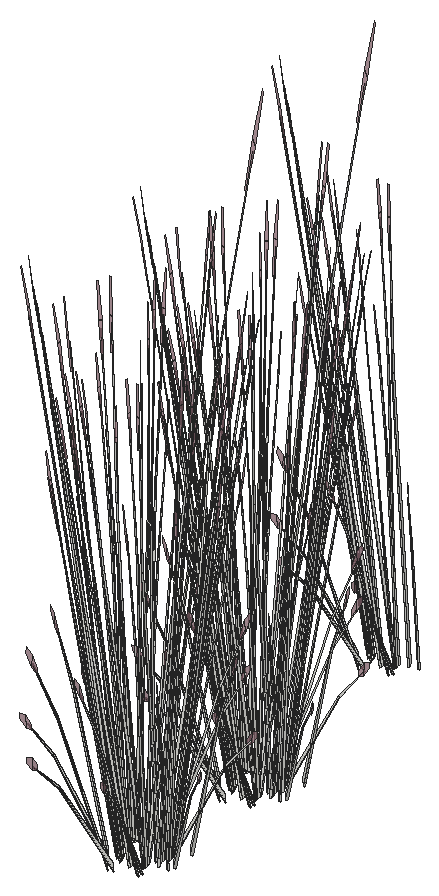
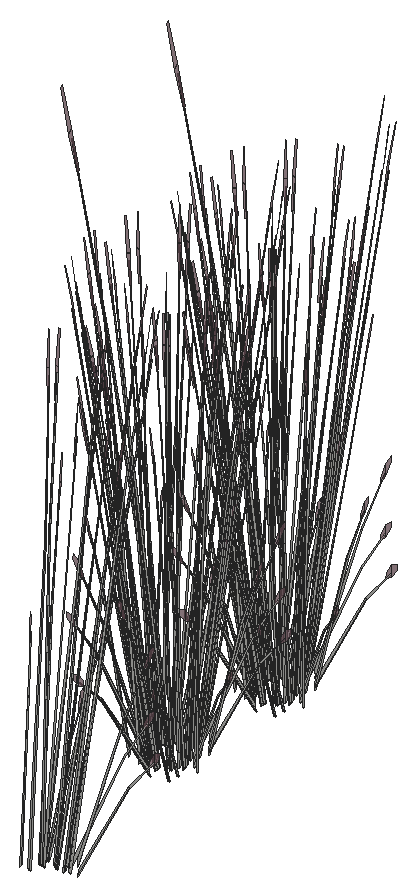
# SketchUp Ruby script. Lengths in inches.
U = 1.inch
M = Sketchup.active_model
def pt(a) = Geom::Point3d.new(a.map { |v| v * U })
def face(e, loops, mat)
  f = e.add_face(loops[0].map { |a| pt(a) })
  loops[1..].each { |l| e.add_face(l.map { |a| pt(a) }).erase! }
  f.material = f.back_material = mat if mat
  f
end
# faces: each face lists its corners as indices into pts; further lists are holes
def faces(e, pts, list, mat = nil) = list.each { |f| face(e, (f[0].is_a?(Array) ? f : [f]).map { |l| l.map { |i| pts[i] } }, mat) }
# xy, xz, yz: faces in a plane at the given z, y or x. An outline is a flat list of corners, or four numbers for a rectangle; further outlines are holes
def ring(l) = l.size == 4 ? [[l[0], l[1]], [l[2], l[1]], [l[2], l[3]], [l[0], l[3]]] : l.each_slice(2).to_a
def flat(e, list, mat, &to3) = list.each { |f| face(e, (f[0].is_a?(Array) ? f : [f]).map { |l| ring(l).map { |u, v| to3.(u, v) } }, mat) }
def xy(e, z, list, mat = nil) = flat(e, list, mat) { |x, y| [x, y, z] }
def xz(e, y, list, mat = nil) = flat(e, list, mat) { |x, z| [x, y, z] }
def yz(e, x, list, mat = nil) = flat(e, list, mat) { |y, z| [x, y, z] }
def lines(e, pts, list) = list.each { |a, b| e.add_line(pt(pts[a]), pt(pts[b])) }
# prism: a flat outline (further loops are holes) pulled along v
def prism(e, loops, v, mat = nil)
  f = face(e, loops, mat); d = Geom::Vector3d.new(v.map { |x| x * U })
  f.pushpull(f.normal.samedirection?(d) ? d.length : -d.length)
end
def box(e, o, s, mat = nil) = prism(e, [[o, [o[0] + s[0], o[1], o[2]], [o[0] + s[0], o[1] + s[1], o[2]], [o[0], o[1] + s[1], o[2]]]], [0, 0, s[2]], mat)
def at(x, y, z, deg = 0) = Geom::Transformation.translation(pt([x, y, z])) * Geom::Transformation.rotation(ORIGIN, Z_AXIS, deg.degrees)
def axes(o, x, y, z) = Geom::Transformation.new([*x, 0, *y, 0, *z, 0, *pt(o).to_a, 1])
def part(name) = M.definitions.add(name)
# library, detail: a bought-in or finely detailed component or shape, given as its bounding box
def library(name, o, s) = part(name).tap { |d| box(d.entities, o, s) }
def detail(e, o, s) = box(e.add_group.entities, o, s)
def put(e, d, t, mat = nil) = e.add_instance(d, t).tap { |i| i.material = mat if mat }
def group(e, t, mat = nil) = e.add_group.tap { |g| g.transformation = t; g.material = mat if mat }.entities
root = M.entities
M.materials.add("LightPink_Translucent").color = [144, 107, 117]
M.materials["LightPink_Translucent"].alpha = 0.75
c1 = part("blade")
p = [[2.15,0.21,22],[0,0.17,0],[0.09,0.45,0],[2.18,0.31,22],[2.29,0.31,22],[0.38,0.45,0],
  [2.48,0.24,33],[2.49,0.24,33],[2.48,0.22,33]]
faces(c1.entities,p,[[0,1,2,3],[4,5,2,3],[6,3,4,7],[8,0,3,6]])
c2 = part("seeds")
p = [[0.3,-0.1,1.38],[-0.01,-0.03,1.59],[-0.01,-0.03,0.03],[0.14,-0.07,-0.07],[0.29,-0.03,3],[0.15,0.01,3.11]]
faces(c2.entities,p,[[0,1,2,3],[1,0,4,5]],"LightPink_Translucent")
c3 = part("blade with seeds")
put(c3.entities,c1,at(0,0,0))
put(c3.entities,c2,axes([2.4,0.25,30.99],[1.5799,-0.05474,1.17369],[-0.12525,1.92788,0.29478],[-0.07173,-0.02425,1.56792]))
put(root,c3,axes([401.89,8.58,4.72],[-0.05398,-0.06539,1.74944],[-0.36026,0.04145,-0.27667],[-0.0575,-0.15639,0.14031]))
put(root,c3,axes([403.51,9.38,4.72],[-0.00341,-0.09282,1.74944],[-0.28775,-0.26825,-0.27667],[0.04449,-0.16261,0.14031]))
put(root,c3,axes([403.43,9.05,4.71],[-0.03584,0.03562,1.77383],[-0.35118,-0.12018,-0.16761],[-0.01271,-0.15545,0.31391]))
put(root,c3,axes([401.52,8.37,4.71],[-0.00658,0.0559,1.77383],[-0.32474,0.20287,-0.16761],[-0.09556,-0.1037,0.31391]))
put(root,c3,axes([401.45,9.36,5.09],[0.39316,-0.11987,0.53763],[0.06823,0.47021,0.4433],[-0.09247,-0.13858,1.11249]))
put(root,c3,axes([402.34,9.45,4.73],[0.34777,0.12192,0.48003],[-0.11892,0.40083,0.3958],[-0.0209,-0.15763,0.9933]))
put(root,c3,axes([402.4375,9.59,5.03],[-0.34538,0.21713,-0.1216],[-0.16972,-0.38536,-0.67495],[-0.04557,-0.16239,1.02557]))
put(root,c3,axes([403.15,10.08,5.03],[-0.3879,-0.02311,-0.1216],[0.0106,-0.43749,-0.67495],[0.02694,-0.1685,1.02557]))
put(root,c3,axes([402.43,9.42,4.73],[0.26007,-0.1585,0.0643],[0.12729,0.28902,0.50621],[-0.02512,-0.1274,0.77189]))
put(root,c3,axes([401.54,9.46,4.73],[0.16041,-0.29625,0.0643],[0.22843,0.17248,0.50621],[-0.07385,-0.09498,0.77189]))
put(root,c3,axes([402.33,9.74,5.05],[-0.1064,0.35863,0.35414],[-0.31043,-0.1046,-0.4572],[-0.02846,-0.14439,0.87481]))
put(root,c3,axes([403.125,9.89,4.73],[0.25132,0.3182,0.48003],[-0.2669,0.27442,0.3958],[0.04636,-0.14929,0.9933]))
put(root,c3,axes([401.61,9.43,5.43],[-0.23555,0.44708,-0.13619],[-0.34112,-0.25757,-0.75594],[-0.11858,-0.12631,1.14864]))
put(root,c3,axes([403.22,9.92,4.73],[0.29004,0.02173,0.0643],[-0.00795,0.32812,0.50621],[0.03035,-0.12569,0.77189]))
put(root,c3,axes([403,10.14,5.05],[-0.23881,0.24554,0.35414],[-0.22606,-0.28036,-0.4572],[0.0344,-0.14245,0.87481]))
put(root,c3,axes([400.71,9.3,4.72],[-0.07594,-0.00329,1.74944],[-0.24177,0.32918,-0.27667],[-0.129,-0.06726,0.14031]))
put(root,c3,axes([403.58,10.9375,5.03],[-0.32648,-0.25715,-0.1216],[0.18809,-0.3724,-0.67495],[0.09224,-0.12945,1.02557]))
put(root,c3,axes([401.59,9.8,5.05],[0.05451,0.37564,0.35414],[-0.31161,0.09919,-0.4572],[-0.0837,-0.10765,0.87481]))
put(root,c3,axes([400.65,10.04,5.09],[0.29147,-0.34417,0.53763],[0.25138,0.3655,0.4433],[-0.13675,-0.06349,1.11249]))
put(root,c3,axes([404.38,10.83,4.71],[-0.0461,-0.00354,1.77383],[-0.19143,-0.37951,-0.16761],[0.07688,-0.12478,0.31391]))
put(root,c3,axes([400.78,10.04,4.73],[0.01777,-0.35463,0.0643],[0.26836,0.00972,0.50621],[-0.1028,-0.03711,0.77189]))
put(root,c3,axes([403.42,10.9,5.05],[-0.30722,0.06665,0.35414],[-0.08112,-0.381,-0.4572],[0.08804,-0.10234,0.87481]))
put(root,c3,axes([403.7,10.84,4.73],[0.2423,0.19613,0.0643],[-0.14107,0.2793,0.50621],[0.07768,-0.0903,0.77189]))
put(root,c3,axes([403.63,10.76,4.73],[0.08753,0.42921,0.48003],[-0.34336,0.07449,0.3958],[0.1012,-0.10094,0.9933]))
put(root,c3,axes([404.55,11.28,4.72],[0.04898,-0.07104,1.74944],[-0.06269,-0.43574,-0.27667],[0.12289,-0.08262,0.14031]))
put(root,c3,axes([400.42,9.58,4.71],[0.02617,0.04654,1.77383],[-0.12614,0.41836,-0.16761],[-0.12775,0.00303,0.31391]))
put(root,c3,axes([400.97,10.31,5.05],[0.20082,0.29199,0.35414],[-0.2293,0.2764,-0.4572],[-0.1165,-0.04206,0.87481]))
put(root,c3,axes([400.91,10.12,5.03],[-0.0189,0.47427,-0.1216],[-0.35781,-0.01296,-0.67495],[-0.13781,-0.03295,1.02557]))
put(root,c3,axes([403.59,11.94,5.03],[-0.17758,-0.42229,-0.1216],[0.31518,-0.20752,-0.67495],[0.13282,-0.05572,1.02557]))
put(root,c3,axes([403.47,11.81,5.05],[-0.29332,-0.1301,0.35414],[0.08555,-0.37955,-0.4572],[0.11809,-0.0348,0.87481]))
put(root,c3,axes([400.4,11.12,4.73],[0.09971,-0.42522,0.48003],[0.32782,0.1454,0.3958],[-0.12892,0.02555,0.9933]))
put(root,c3,axes([400.37,11.01,4.73],[-0.12963,-0.31798,0.0643],[0.23638,-0.15564,0.50621],[-0.1042,0.03071,0.77189]))
put(root,c3,axes([403.73,11.93,4.73],[0.12963,0.31798,0.0643],[-0.23638,0.15564,0.50621],[0.1042,-0.03071,0.77189]))
put(root,c3,axes([403.71,11.82,4.73],[-0.09971,0.42522,0.48003],[-0.32782,-0.1454,0.3958],[0.12892,-0.02555,0.9933]))
put(root,c3,axes([400.64,11.125,5.05],[0.29332,0.1301,0.35414],[-0.08555,0.37955,-0.4572],[-0.11809,0.0348,0.87481]))
put(root,c3,axes([404.3,13.2,4.71],[-0.03191,-0.04083,1.77383],[0.06981,-0.43764,-0.16761],[0.12571,-0.02796,0.31391]))
put(root,c3,axes([400.14,11.42,4.72],[-0.05763,0.06055,1.74944],[0.0049,0.44239,-0.27667],[-0.13211,0.05753,0.14031]))
put(root,c3,axes([400.51,11,5.03],[0.17758,0.42229,-0.1216],[-0.31518,0.20752,-0.67495],[-0.13282,0.05572,1.02557]))
put(root,c3,axes([403.19,12.82,5.03],[0.0189,-0.47427,-0.1216],[0.35781,0.01296,-0.67495],[0.13781,0.03295,1.02557]))
put(root,c3,axes([403.14,12.63,5.05],[-0.20082,-0.29199,0.35414],[0.2293,-0.2764,-0.4572],[0.1165,0.04206,0.87481]))
put(root,c3,axes([403.5,12.53,4.72],[0.07571,-0.00789,1.74944],[0.20767,-0.36231,-0.27667],[0.13467,0.04783,0.14031]))
put(root,c3,axes([400.47,12.18,4.73],[-0.08753,-0.42921,0.48003],[0.34336,-0.07449,0.3958],[-0.1012,0.10094,0.9933]))
put(root,c3,axes([400.41,12.1,4.73],[-0.2423,-0.19613,0.0643],[0.14107,-0.2793,0.50621],[-0.07768,0.0903,0.77189]))
put(root,c3,axes([400.6875,12.04,5.05],[0.30722,-0.06665,0.35414],[0.08112,0.381,-0.4572],[-0.08804,0.10234,0.87481]))
put(root,c3,axes([399.5,11.87,4.71],[0.04504,0.01251,1.77383],[0.13934,0.41205,-0.16761],[-0.0922,0.10815,0.31391]))
put(root,c3,axes([403.32,12.9,4.73],[-0.01777,0.35463,0.0643],[-0.26836,-0.00972,0.50621],[0.1028,0.03711,0.77189]))
put(root,c3,axes([403.34,12.79,4.73],[-0.26024,0.30729,0.48003],[-0.22444,-0.32634,0.3958],[0.1221,0.05668,0.9933]))
put(root,c3,axes([399.99,13.12,5.65],[0.31145,0.12449,-0.06488],[-0.0958,0.38314,-0.29416],[-0.05094,0.05817,0.97024]))
put(root,c3,axes([402.52,13.14,5.05],[-0.05451,-0.37564,0.35414],[0.31161,-0.09919,-0.4572],[0.0837,0.10765,0.87481]))
put(root,c3,axes([402.72,10.98,4.47],[-0.30498,-0.24231,1.38283],[0.32203,-0.37727,0.59665],[0.0984,0.22736,1.33663]))
put(root,c3,axes([400.53,12,5.03],[0.32648,0.25715,-0.1216],[-0.18809,0.3724,-0.67495],[-0.09224,0.12945,1.02557]))
put(root,c3,axes([402.49,13.34,5.03],[0.21031,-0.39918,-0.1216],[0.30457,0.22997,-0.67495],[0.10587,0.11278,1.02557]))
put(root,c3,axes([401.1,12.8,5.05],[0.23881,-0.24554,0.35414],[0.22606,0.28036,-0.4572],[-0.0344,0.14245,0.87481]))
put(root,c3,axes([402.21,13.67,4.71],[0.00104,-0.05646,1.77383],[0.30246,-0.2491,-0.16761],[0.10506,0.08891,0.31391]))
put(root,c3,axes([400.88,13.02,4.73],[-0.29004,-0.02173,0.0643],[0.00795,-0.32812,0.50621],[-0.03035,0.12569,0.77189]))
put(root,c3,axes([400.98,13.05,4.73],[-0.25132,-0.3182,0.48003],[0.2669,-0.27442,0.3958],[-0.04636,0.14929,0.9933]))
put(root,c3,axes([401.77,13.2,5.05],[0.1064,-0.35863,0.35414],[0.31043,0.1046,-0.4572],[0.02846,0.14439,0.87481]))
put(root,c3,axes([402.56,13.48,4.73],[-0.16041,0.29625,0.0643],[-0.22843,-0.17248,0.50621],[0.07385,0.09498,0.77189]))
put(root,c3,axes([402.1875,14.48,5.65],[0.2439,-0.26754,-0.06488],[0.22348,0.29302,-0.29416],[0.01573,0.08303,0.97024]))
put(root,c3,axes([402.63,13.4,4.73],[-0.35104,0.10702,0.48003],[-0.06092,-0.41983,0.3958],[0.08256,0.12373,0.9933]))
put(root,c3,axes([401.67,13.53,4.73],[-0.26007,0.1585,0.0643],[-0.12729,-0.28902,0.50621],[0.02512,0.1274,0.77189]))
put(root,c3,axes([400.15,13.07,4.72],[-0.00877,0.09229,1.74944],[0.24897,0.32105,-0.27667],[-0.06518,0.15182,0.14031]))
put(root,c3,axes([400.95,12.86,5.4],[0.3879,0.02311,-0.13498],[-0.0106,0.43749,-0.74919],[-0.02694,0.1685,1.13838]))
put(root,c3,axes([401.67,13.35,5.03],[0.34538,-0.21713,-0.1216],[0.16972,0.38536,-0.67495],[0.04557,0.16239,1.02557]))
put(root,c3,axes([401.77,13.49,5.0625],[-0.34777,-0.12192,0.53283],[0.11892,-0.40083,0.43934],[0.0209,0.15763,1.10256]))
put(root,c3,axes([401.89,19.52,4.72],[-0.05398,-0.06539,1.74944],[-0.36026,0.04145,-0.27667],[-0.0575,-0.15639,0.14031]))
put(root,c3,axes([400.125,14.02,4.71],[0.04004,-0.02816,1.77383],[0.33095,0.18728,-0.16761],[-0.00778,0.15594,0.31391]))
put(root,c3,axes([403.51,20.33,4.72],[-0.00341,-0.09282,1.74944],[-0.28775,-0.26825,-0.27667],[0.04449,-0.16261,0.14031]))
put(root,c3,axes([403.43,19.99,4.71],[-0.03584,0.03562,1.77383],[-0.35118,-0.12018,-0.16761],[-0.01271,-0.15545,0.31391]))
put(root,c3,axes([401.58,14.21,4.72],[0.04474,0.0751,1.74944],[0.36104,0.0295,-0.27667],[0.03631,0.16562,0.14031]))
put(root,c3,axes([401.52,19.31,4.71],[-0.00658,0.0559,1.77383],[-0.32474,0.20287,-0.16761],[-0.09556,-0.1037,0.31391]))
put(root,c3,axes([401.45,20.3,5.09],[0.39316,-0.11987,0.53763],[0.06823,0.47021,0.4433],[-0.09247,-0.13858,1.11249]))
put(root,c3,axes([402.34,20.39,4.73],[0.34777,0.12192,0.48003],[-0.11892,0.40083,0.3958],[-0.0209,-0.15763,0.9933]))
put(root,c3,axes([402.4375,20.53,5.03],[-0.34538,0.21713,-0.1216],[-0.16972,-0.38536,-0.67495],[-0.04557,-0.16239,1.02557]))
put(root,c3,axes([403.15,21.02,5.03],[-0.3879,-0.02311,-0.1216],[0.0106,-0.43749,-0.67495],[0.02694,-0.1685,1.02557]))
put(root,c3,axes([402.43,20.36,4.73],[0.26007,-0.1585,0.0643],[0.12729,0.28902,0.50621],[-0.02512,-0.1274,0.77189]))
put(root,c3,axes([401.54,20.4,4.73],[0.16041,-0.29625,0.0643],[0.22843,0.17248,0.50621],[-0.07385,-0.09498,0.77189]))
put(root,c3,axes([402.33,20.68,5.05],[-0.1064,0.35863,0.35414],[-0.31043,-0.1046,-0.4572],[-0.02846,-0.14439,0.87481]))
put(root,c3,axes([403.125,20.84,4.73],[0.25132,0.3182,0.48003],[-0.2669,0.27442,0.3958],[0.04636,-0.14929,0.9933]))
put(root,c3,axes([401.61,20.375,5.43],[-0.23555,0.44708,-0.13619],[-0.34112,-0.25757,-0.75594],[-0.11858,-0.12631,1.14864]))
put(root,c3,axes([403.22,20.87,4.73],[0.29004,0.02173,0.0643],[-0.00795,0.32812,0.50621],[0.03035,-0.12569,0.77189]))
put(root,c3,axes([403,21.09,5.05],[-0.23881,0.24554,0.35414],[-0.22606,-0.28036,-0.4572],[0.0344,-0.14245,0.87481]))
put(root,c3,axes([400.71,20.24,4.72],[-0.07594,-0.00329,1.74944],[-0.24177,0.32918,-0.27667],[-0.129,-0.06726,0.14031]))
put(root,c3,axes([403.58,21.88,5.03],[-0.32648,-0.25715,-0.1216],[0.18809,-0.3724,-0.67495],[0.09224,-0.12945,1.02557]))
put(root,c3,axes([401.59,20.74,5.05],[0.05451,0.37564,0.35414],[-0.31161,0.09919,-0.4572],[-0.0837,-0.10765,0.87481]))
put(root,c3,axes([400.65,20.99,5.09],[0.29147,-0.34417,0.53763],[0.25138,0.3655,0.4433],[-0.13675,-0.06349,1.11249]))
put(root,c3,axes([404.38,21.77,4.71],[-0.0461,-0.00354,1.77383],[-0.19143,-0.37951,-0.16761],[0.07688,-0.12478,0.31391]))
put(root,c3,axes([400.78,20.99,4.73],[0.01777,-0.35463,0.0643],[0.26836,0.00972,0.50621],[-0.1028,-0.03711,0.77189]))
put(root,c3,axes([403.42,21.85,5.05],[-0.30722,0.06665,0.35414],[-0.08112,-0.381,-0.4572],[0.08804,-0.10234,0.87481]))
put(root,c3,axes([403.7,21.79,4.73],[0.2423,0.19613,0.0643],[-0.14107,0.2793,0.50621],[0.07768,-0.0903,0.77189]))
put(root,c3,axes([403.63,21.71,4.73],[0.08753,0.42921,0.48003],[-0.34336,0.07449,0.3958],[0.1012,-0.10094,0.9933]))
put(root,c3,axes([404.55,22.22,4.72],[0.04898,-0.07104,1.74944],[-0.06269,-0.43574,-0.27667],[0.12289,-0.08262,0.14031]))
put(root,c3,axes([400.42,20.52,4.71],[0.02617,0.04654,1.77383],[-0.12614,0.41836,-0.16761],[-0.12775,0.00303,0.31391]))
put(root,c3,axes([400.97,21.25,5.05],[0.20082,0.29199,0.35414],[-0.2293,0.2764,-0.4572],[-0.1165,-0.04206,0.87481]))
put(root,c3,axes([400.91,21.07,5.03],[-0.0189,0.47427,-0.1216],[-0.35781,-0.01296,-0.67495],[-0.13781,-0.03295,1.02557]))
put(root,c3,axes([403.59,22.89,5.03],[-0.17758,-0.42229,-0.1216],[0.31518,-0.20752,-0.67495],[0.13282,-0.05572,1.02557]))
put(root,c3,axes([403.47,22.76,5.05],[-0.29332,-0.1301,0.35414],[0.08555,-0.37955,-0.4572],[0.11809,-0.0348,0.87481]))
put(root,c3,axes([400.4,22.07,4.73],[0.09971,-0.42522,0.48003],[0.32782,0.1454,0.3958],[-0.12892,0.02555,0.9933]))
put(root,c3,axes([400.37,21.95,4.73],[-0.12963,-0.31798,0.0643],[0.23638,-0.15564,0.50621],[-0.1042,0.03071,0.77189]))
put(root,c3,axes([403.73,22.875,4.73],[0.12963,0.31798,0.0643],[-0.23638,0.15564,0.50621],[0.1042,-0.03071,0.77189]))
put(root,c3,axes([403.71,22.76,4.73],[-0.09971,0.42522,0.48003],[-0.32782,-0.1454,0.3958],[0.12892,-0.02555,0.9933]))
put(root,c3,axes([400.64,22.07,5.05],[0.29332,0.1301,0.35414],[-0.08555,0.37955,-0.4572],[-0.11809,0.0348,0.87481]))
put(root,c3,axes([404.3,24.14,4.71],[-0.03191,-0.04083,1.77383],[0.06981,-0.43764,-0.16761],[0.12571,-0.02796,0.31391]))
put(root,c3,axes([400.14,22.37,4.72],[-0.05763,0.06055,1.74944],[0.0049,0.44239,-0.27667],[-0.13211,0.05753,0.14031]))
put(root,c3,axes([400.51,21.94,5.03],[0.17758,0.42229,-0.1216],[-0.31518,0.20752,-0.67495],[-0.13282,0.05572,1.02557]))
put(root,c3,axes([403.19,23.76,5.03],[0.0189,-0.47427,-0.1216],[0.35781,0.01296,-0.67495],[0.13781,0.03295,1.02557]))
put(root,c3,axes([403.14,23.58,5.05],[-0.20082,-0.29199,0.35414],[0.2293,-0.2764,-0.4572],[0.1165,0.04206,0.87481]))
put(root,c3,axes([403.5,23.48,4.72],[0.07571,-0.00789,1.74944],[0.20767,-0.36231,-0.27667],[0.13467,0.04783,0.14031]))
put(root,c3,axes([400.47,23.125,4.73],[-0.08753,-0.42921,0.48003],[0.34336,-0.07449,0.3958],[-0.1012,0.10094,0.9933]))
put(root,c3,axes([400.41,23.04,4.73],[-0.2423,-0.19613,0.0643],[0.14107,-0.2793,0.50621],[-0.07768,0.0903,0.77189]))
put(root,c3,axes([400.6875,22.98,5.05],[0.30722,-0.06665,0.35414],[0.08112,0.381,-0.4572],[-0.08804,0.10234,0.87481]))
put(root,c3,axes([399.5,22.8125,4.71],[0.04504,0.01251,1.77383],[0.13934,0.41205,-0.16761],[-0.0922,0.10815,0.31391]))
put(root,c3,axes([403.32,23.84,4.73],[-0.01777,0.35463,0.0643],[-0.26836,-0.00972,0.50621],[0.1028,0.03711,0.77189]))
put(root,c3,axes([403.34,23.73,4.73],[-0.26024,0.30729,0.48003],[-0.22444,-0.32634,0.3958],[0.1221,0.05668,0.9933]))
put(root,c3,axes([399.99,24.0625,5.65],[0.31145,0.12449,-0.06488],[-0.0958,0.38314,-0.29416],[-0.05094,0.05817,0.97024]))
put(root,c3,axes([402.52,24.09,5.05],[-0.05451,-0.37564,0.35414],[0.31161,-0.09919,-0.4572],[0.0837,0.10765,0.87481]))
put(root,c3,axes([402.72,21.92,4.47],[-0.30498,-0.24231,1.38283],[0.32203,-0.37727,0.59665],[0.0984,0.22736,1.33663]))
put(root,c3,axes([400.53,22.95,5.03],[0.32648,0.25715,-0.1216],[-0.18809,0.3724,-0.67495],[-0.09224,0.12945,1.02557]))
put(root,c3,axes([402.49,24.28,5.03],[0.21031,-0.39918,-0.1216],[0.30457,0.22997,-0.67495],[0.10587,0.11278,1.02557]))
put(root,c3,axes([401.1,23.74,5.05],[0.23881,-0.24554,0.35414],[0.22606,0.28036,-0.4572],[-0.0344,0.14245,0.87481]))
put(root,c3,axes([402.21,24.61,4.71],[0.00104,-0.05646,1.77383],[0.30246,-0.2491,-0.16761],[0.10506,0.08891,0.31391]))
put(root,c3,axes([400.88,23.96,4.73],[-0.29004,-0.02173,0.0643],[0.00795,-0.32812,0.50621],[-0.03035,0.12569,0.77189]))
put(root,c3,axes([400.98,23.99,4.73],[-0.25132,-0.3182,0.48003],[0.2669,-0.27442,0.3958],[-0.04636,0.14929,0.9933]))
put(root,c3,axes([401.77,24.14,5.05],[0.1064,-0.35863,0.35414],[0.31043,0.1046,-0.4572],[0.02846,0.14439,0.87481]))
put(root,c3,axes([402.56,24.43,4.73],[-0.16041,0.29625,0.0643],[-0.22843,-0.17248,0.50621],[0.07385,0.09498,0.77189]))
put(root,c3,axes([402.1875,25.42,5.65],[0.2439,-0.26754,-0.06488],[0.22348,0.29302,-0.29416],[0.01573,0.08303,0.97024]))
put(root,c3,axes([402.63,24.34,4.73],[-0.35104,0.10702,0.48003],[-0.06092,-0.41983,0.3958],[0.08256,0.12373,0.9933]))
put(root,c3,axes([401.67,24.47,4.73],[-0.26007,0.1585,0.0643],[-0.12729,-0.28902,0.50621],[0.02512,0.1274,0.77189]))
put(root,c3,axes([400.15,24.02,4.72],[-0.00877,0.09229,1.74944],[0.24897,0.32105,-0.27667],[-0.06518,0.15182,0.14031]))
put(root,c3,axes([400.95,23.81,5.4],[0.3879,0.02311,-0.13498],[-0.0106,0.43749,-0.74919],[-0.02694,0.1685,1.13838]))
put(root,c3,axes([401.67,24.3,5.03],[0.34538,-0.21713,-0.1216],[0.16972,0.38536,-0.67495],[0.04557,0.16239,1.02557]))
put(root,c3,axes([401.77,24.4375,5.0625],[-0.34777,-0.12192,0.53283],[0.11892,-0.40083,0.43934],[0.0209,0.15763,1.10256]))
put(root,c3,axes([400.125,24.96,4.71],[0.04004,-0.02816,1.77383],[0.33095,0.18728,-0.16761],[-0.00778,0.15594,0.31391]))
put(root,c3,axes([401.58,25.16,4.72],[0.04474,0.0751,1.74944],[0.36104,0.0295,-0.27667],[0.03631,0.16562,0.14031]))
put(root,c3,axes([398.29,37.57,4.72],[-0.05398,-0.06539,1.74944],[-0.36026,0.04145,-0.27667],[-0.0575,-0.15639,0.14031]))
put(root,c3,axes([399.91,38.37,4.72],[-0.00341,-0.09282,1.74944],[-0.28775,-0.26825,-0.27667],[0.04449,-0.16261,0.14031]))
put(root,c3,axes([399.83,38.04,4.71],[-0.03584,0.03562,1.77383],[-0.35118,-0.12018,-0.16761],[-0.01271,-0.15545,0.31391]))
put(root,c3,axes([397.92,37.36,4.71],[-0.00658,0.0559,1.77383],[-0.32474,0.20287,-0.16761],[-0.09556,-0.1037,0.31391]))
put(root,c3,axes([397.85,38.35,5.09],[0.39316,-0.11987,0.53763],[0.06823,0.47021,0.4433],[-0.09247,-0.13858,1.11249]))
put(root,c3,axes([398.74,38.4375,4.73],[0.34777,0.12192,0.48003],[-0.11892,0.40083,0.3958],[-0.0209,-0.15763,0.9933]))
put(root,c3,axes([398.84,38.58,5.03],[-0.34538,0.21713,-0.1216],[-0.16972,-0.38536,-0.67495],[-0.04557,-0.16239,1.02557]))
put(root,c3,axes([399.56,39.07,5.03],[-0.3879,-0.02311,-0.1216],[0.0106,-0.43749,-0.67495],[0.02694,-0.1685,1.02557]))
put(root,c3,axes([398.83,38.41,4.73],[0.26007,-0.1585,0.0643],[0.12729,0.28902,0.50621],[-0.02512,-0.1274,0.77189]))
put(root,c3,axes([397.94,38.45,4.73],[0.16041,-0.29625,0.0643],[0.22843,0.17248,0.50621],[-0.07385,-0.09498,0.77189]))
put(root,c3,axes([398.74,38.73,5.05],[-0.1064,0.35863,0.35414],[-0.31043,-0.1046,-0.4572],[-0.02846,-0.14439,0.87481]))
put(root,c3,axes([399.53,38.88,4.73],[0.25132,0.3182,0.48003],[-0.2669,0.27442,0.3958],[0.04636,-0.14929,0.9933]))
put(root,c3,axes([398.01,38.42,5.43],[-0.23555,0.44708,-0.13619],[-0.34112,-0.25757,-0.75594],[-0.11858,-0.12631,1.14864]))
put(root,c3,axes([399.62,38.91,4.73],[0.29004,0.02173,0.0643],[-0.00795,0.32812,0.50621],[0.03035,-0.12569,0.77189]))
put(root,c3,axes([399.41,39.13,5.05],[-0.23881,0.24554,0.35414],[-0.22606,-0.28036,-0.4572],[0.0344,-0.14245,0.87481]))
put(root,c3,axes([397.11,38.29,4.72],[-0.07594,-0.00329,1.74944],[-0.24177,0.32918,-0.27667],[-0.129,-0.06726,0.14031]))
put(root,c3,axes([399.98,39.93,5.03],[-0.32648,-0.25715,-0.1216],[0.18809,-0.3724,-0.67495],[0.09224,-0.12945,1.02557]))
put(root,c3,axes([397.99,38.79,5.05],[0.05451,0.37564,0.35414],[-0.31161,0.09919,-0.4572],[-0.0837,-0.10765,0.87481]))
put(root,c3,axes([397.06,39.04,5.09],[0.29147,-0.34417,0.53763],[0.25138,0.3655,0.4433],[-0.13675,-0.06349,1.11249]))
put(root,c3,axes([400.78,39.82,4.71],[-0.0461,-0.00354,1.77383],[-0.19143,-0.37951,-0.16761],[0.07688,-0.12478,0.31391]))
